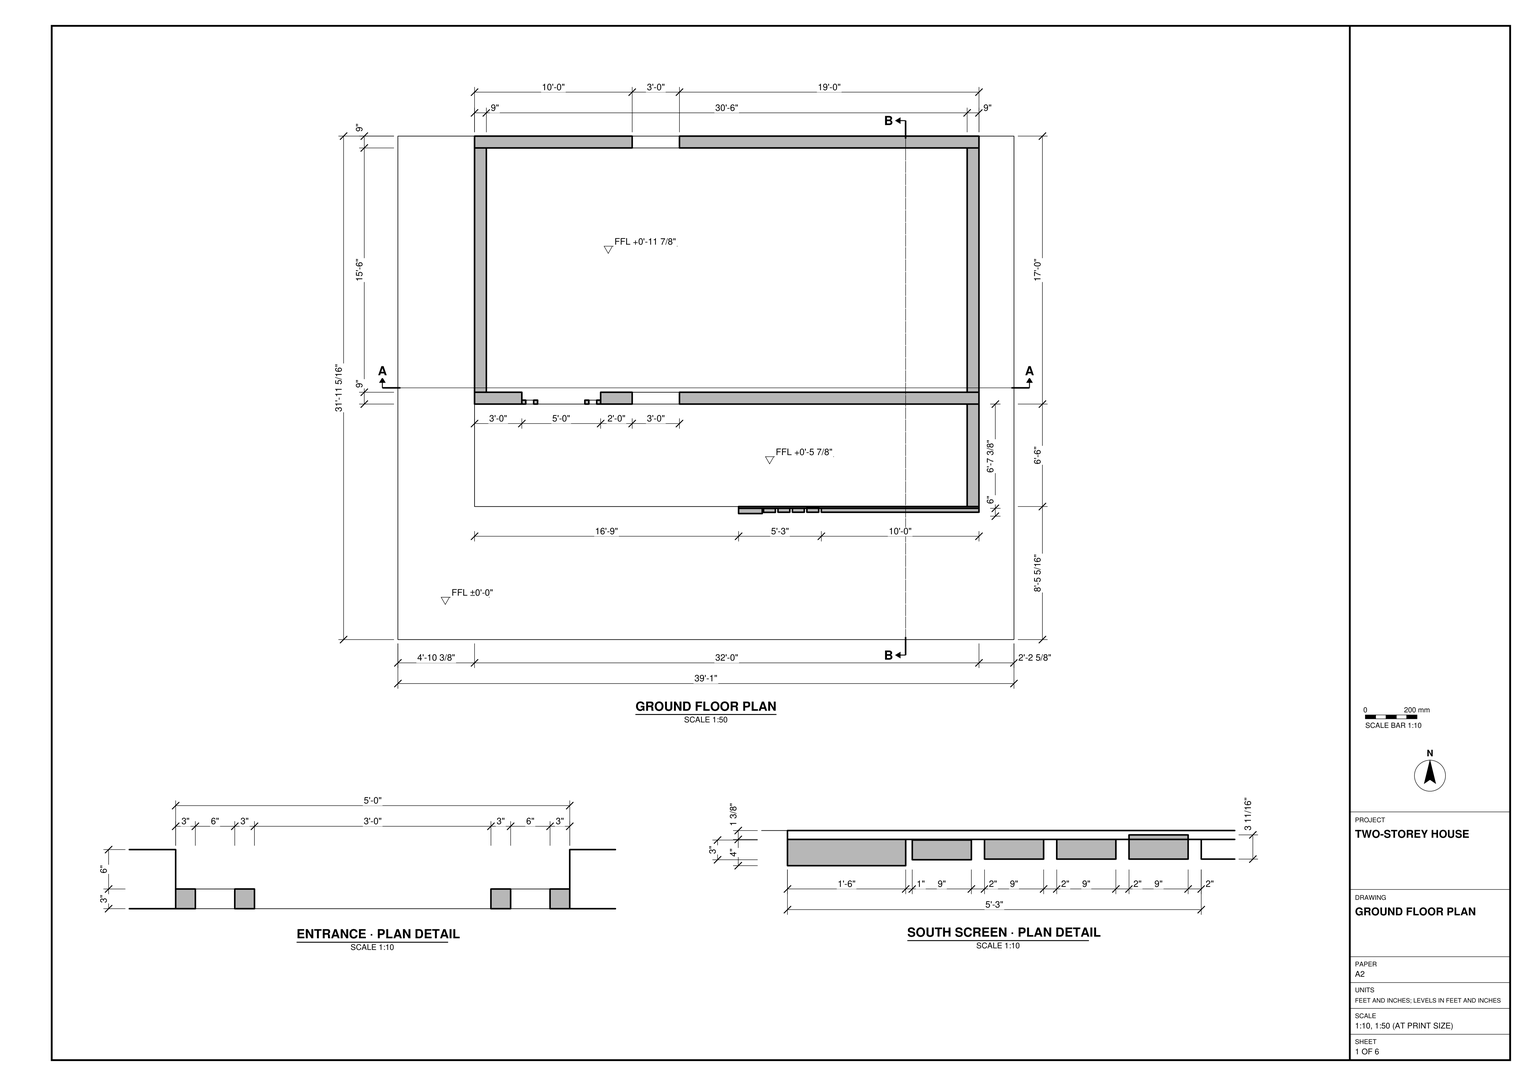
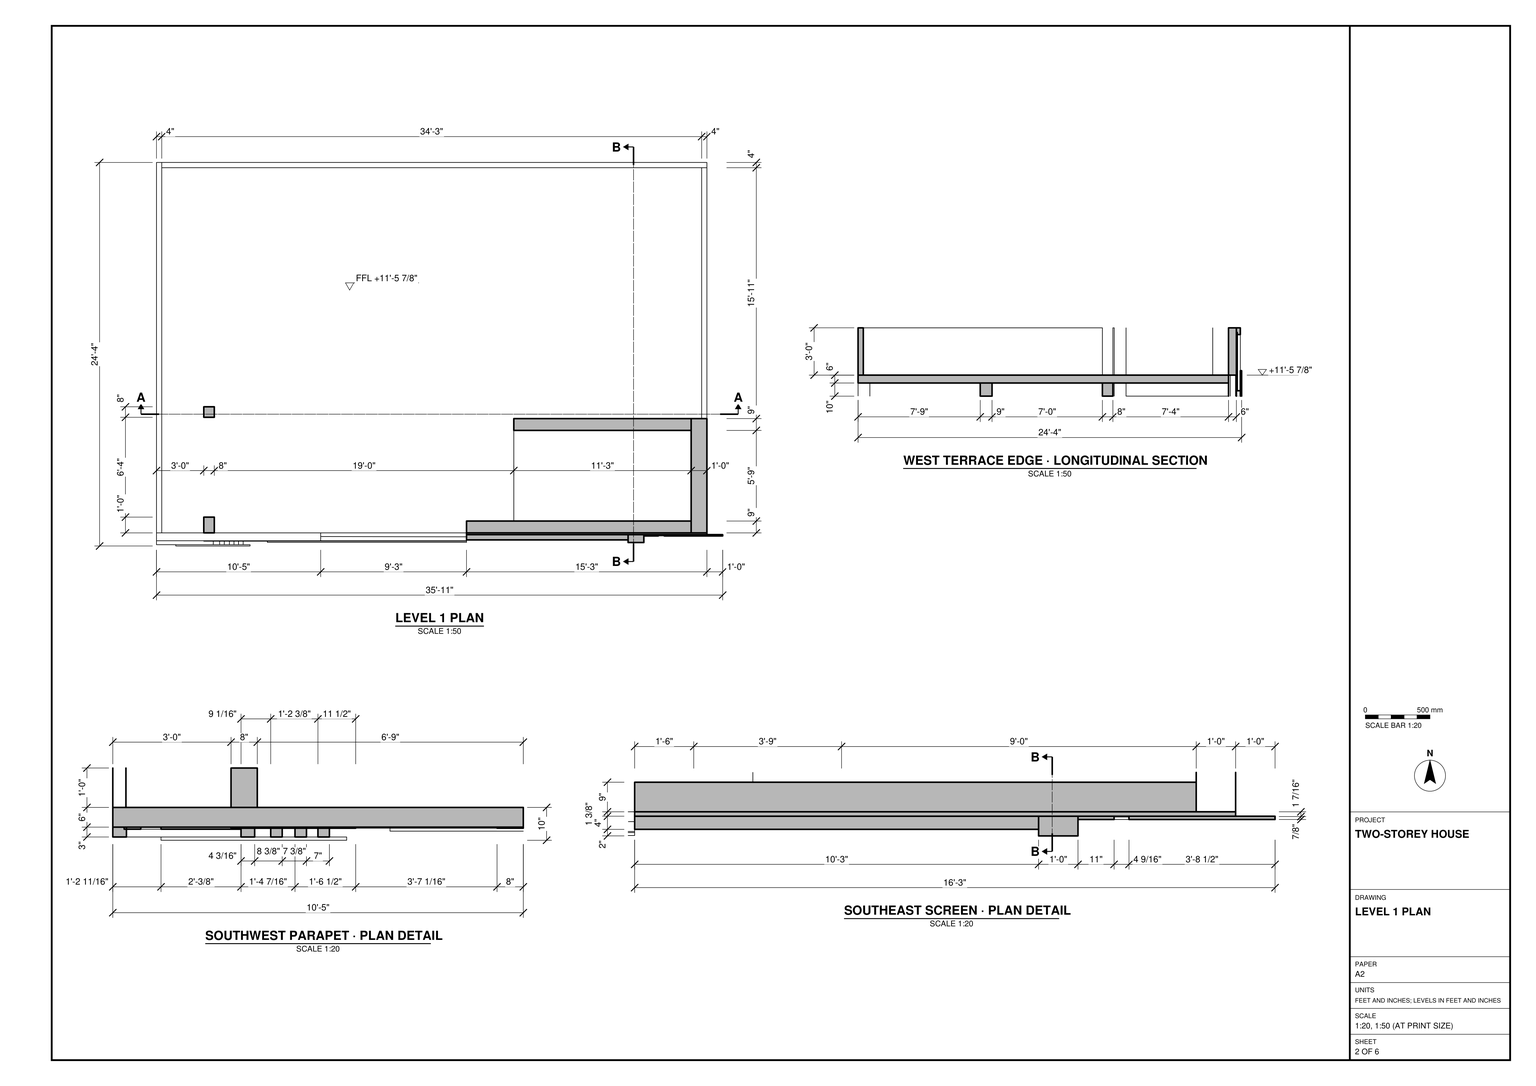
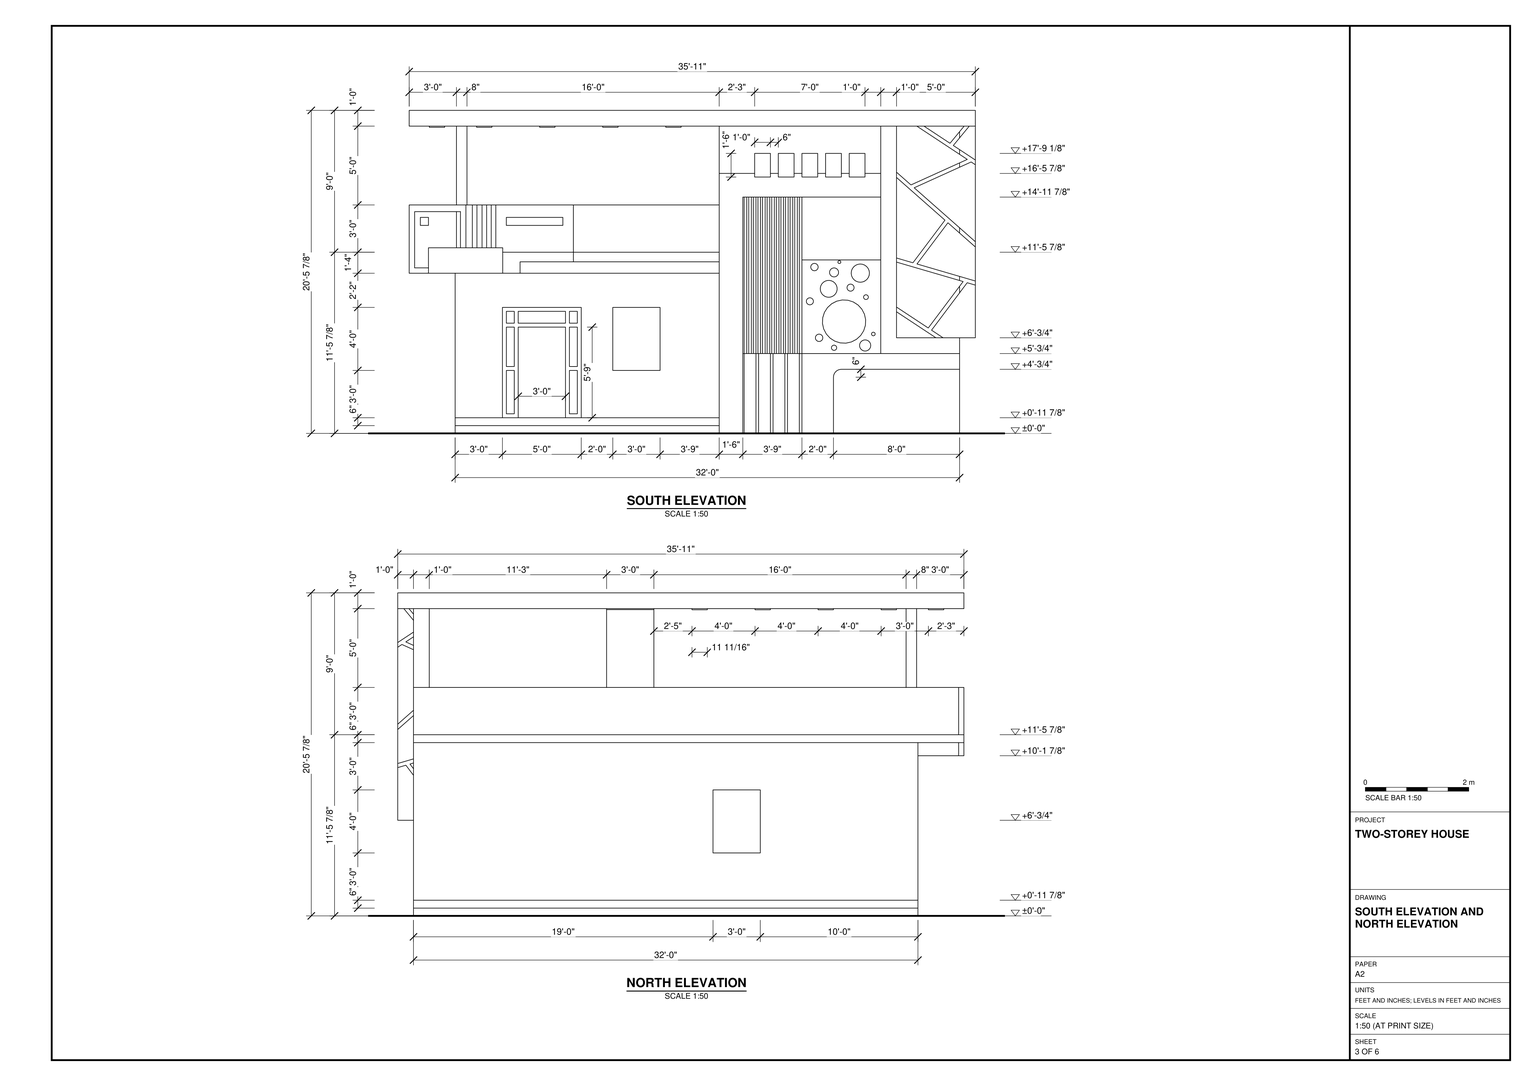
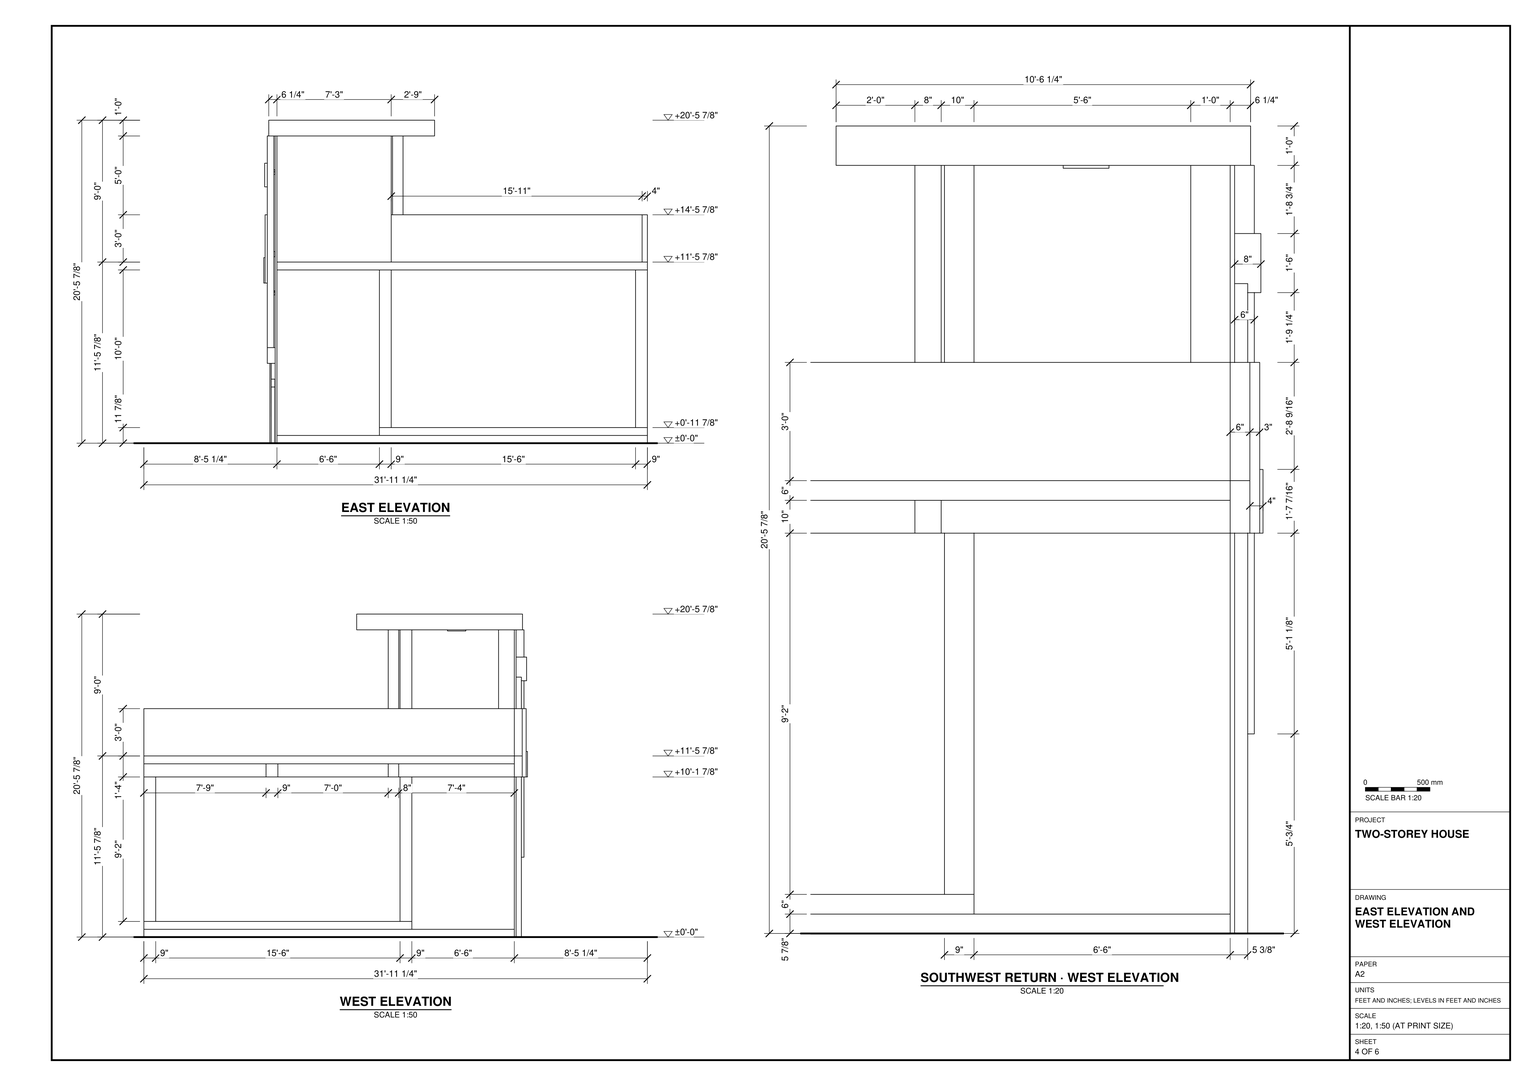
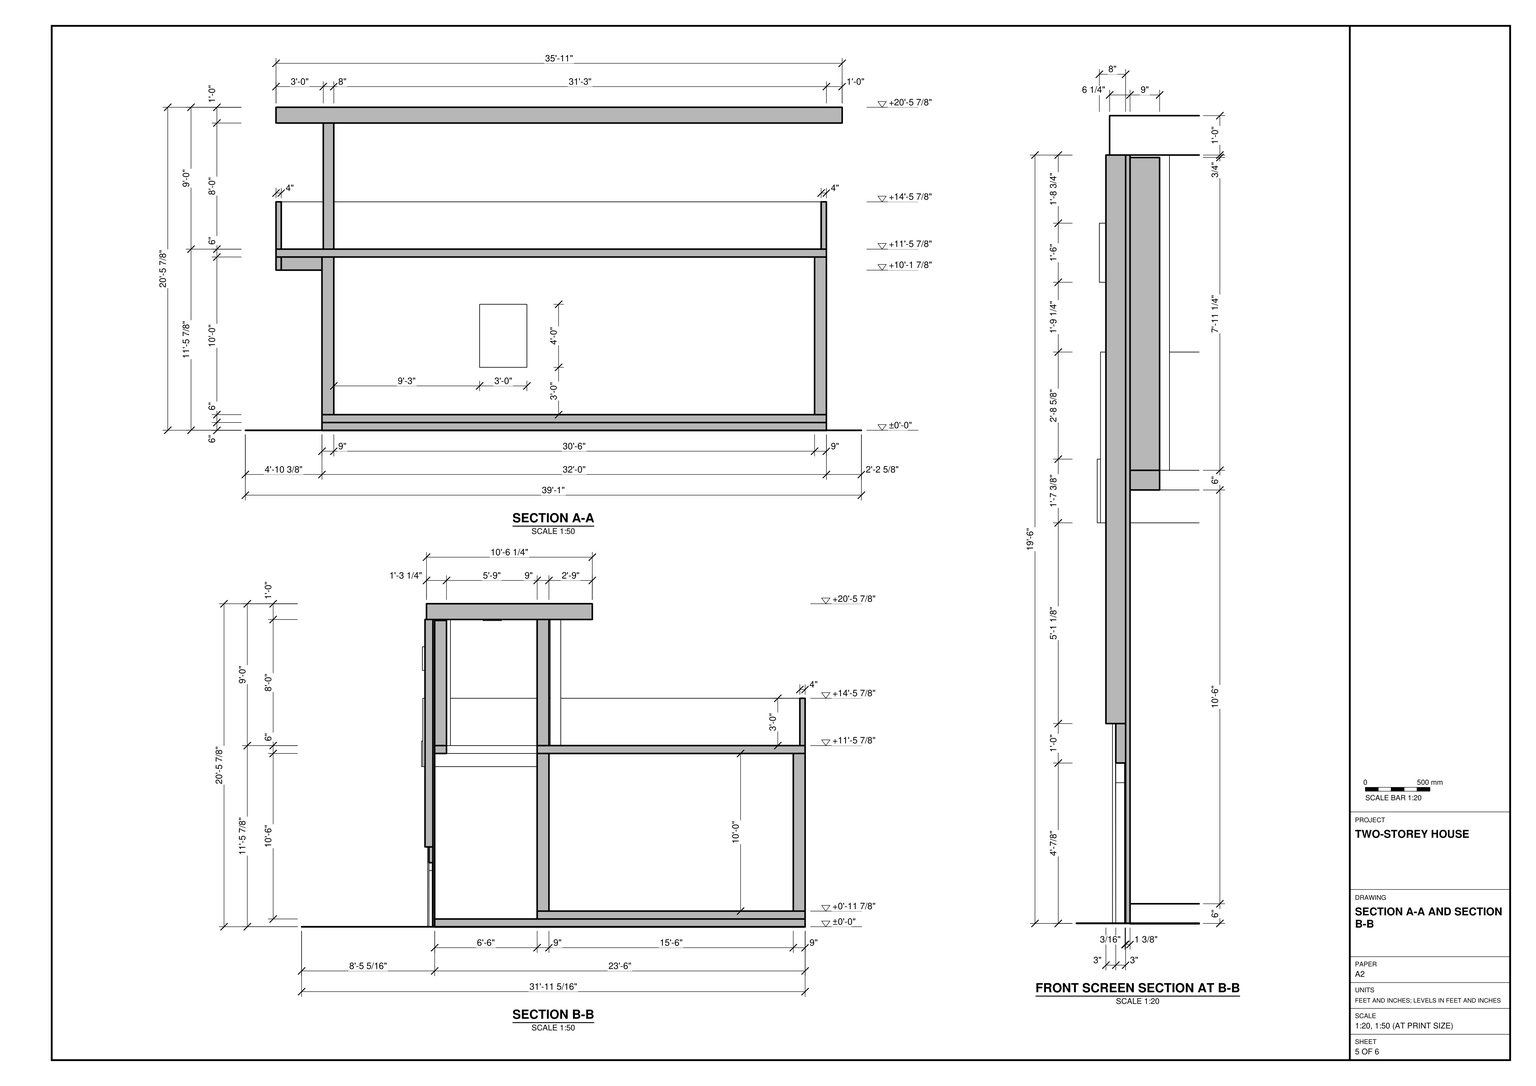
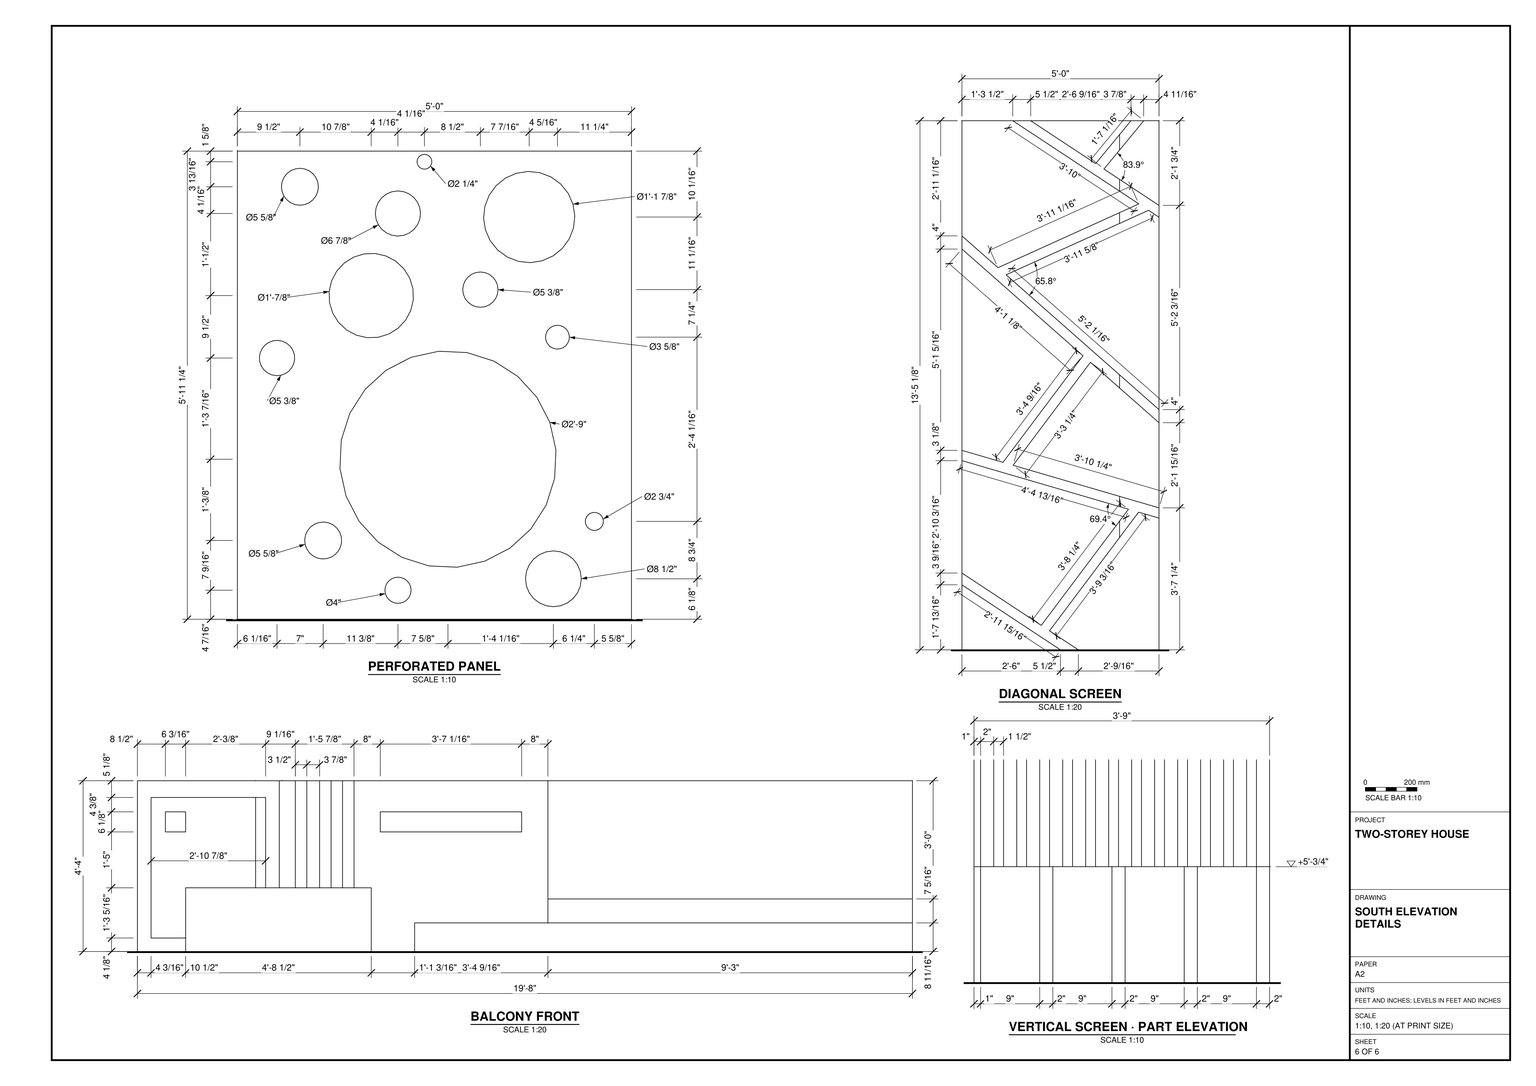
Use task_files/diagram_01.pdf to build the house in SketchUp. Work in feet and inches. Including the base, the model measures 39'-1" along X, 31'-11 5/16" along Y and 20'-6 1/8" along Z. Use ±0'-0" as the ground datum and +11'-5 7/8" as the upper terrace level.

Set out the 32'-0" by 17'-0" ground-floor enclosure on the base with 9" walls. Step up from the base to the south porch at +0'-5 7/8" and then to the interior floor at +0'-11 7/8". Use the entrance detail to frame the doorway, and align the south and north window openings in plan.

Model the projecting terrace slab, its parapets and posts, and the flat roof above. Keep the open space between the parapets and roof as shown in elevation. Use the enlarged plans to set the thickness and spacing of the south screen elements, and the south elevation to place the vertical slats, circular-patterned panel and diagonal end screen.

Keep walls, slabs, roof and individual furniture or joinery pieces in separate groups or components, and use components for repeated parts. Decor and loose items may be any suitable library components. Save one SketchUp model as output_files/two_storey_house_with_covered_terrace_and_south_screens.skp.

# SketchUp Ruby script. Lengths in inches.
U = 1.inch
M = Sketchup.active_model
def pt(a) = Geom::Point3d.new(a.map { |v| v * U })
def face(e, loops, mat)
  f = e.add_face(loops[0].map { |a| pt(a) })
  loops[1..].each { |l| e.add_face(l.map { |a| pt(a) }).erase! }
  f.material = f.back_material = mat if mat
  f
end
# faces: each face lists its corners as indices into pts; further lists are holes
def faces(e, pts, list, mat = nil) = list.each { |f| face(e, (f[0].is_a?(Array) ? f : [f]).map { |l| l.map { |i| pts[i] } }, mat) }
# xy, xz, yz: faces in a plane at the given z, y or x. An outline is a flat list of corners, or four numbers for a rectangle; further outlines are holes
def ring(l) = l.size == 4 ? [[l[0], l[1]], [l[2], l[1]], [l[2], l[3]], [l[0], l[3]]] : l.each_slice(2).to_a
def flat(e, list, mat, &to3) = list.each { |f| face(e, (f[0].is_a?(Array) ? f : [f]).map { |l| ring(l).map { |u, v| to3.(u, v) } }, mat) }
def xy(e, z, list, mat = nil) = flat(e, list, mat) { |x, y| [x, y, z] }
def xz(e, y, list, mat = nil) = flat(e, list, mat) { |x, z| [x, y, z] }
def yz(e, x, list, mat = nil) = flat(e, list, mat) { |y, z| [x, y, z] }
def lines(e, pts, list) = list.each { |a, b| e.add_line(pt(pts[a]), pt(pts[b])) }
# prism: a flat outline (further loops are holes) pulled along v
def prism(e, loops, v, mat = nil)
  f = face(e, loops, mat); d = Geom::Vector3d.new(v.map { |x| x * U })
  f.pushpull(f.normal.samedirection?(d) ? d.length : -d.length)
end
def box(e, o, s, mat = nil) = prism(e, [[o, [o[0] + s[0], o[1], o[2]], [o[0] + s[0], o[1] + s[1], o[2]], [o[0], o[1] + s[1], o[2]]]], [0, 0, s[2]], mat)
def at(x, y, z, deg = 0) = Geom::Transformation.translation(pt([x, y, z])) * Geom::Transformation.rotation(ORIGIN, Z_AXIS, deg.degrees)
def axes(o, x, y, z) = Geom::Transformation.new([*x, 0, *y, 0, *z, 0, *pt(o).to_a, 1])
def part(name) = M.definitions.add(name)
# library, detail: a bought-in or finely detailed component or shape, given as its bounding box
def library(name, o, s) = part(name).tap { |d| box(d.entities, o, s) }
def detail(e, o, s) = box(e.add_group.entities, o, s)
def put(e, d, t, mat = nil) = e.add_instance(d, t).tap { |i| i.material = mat if mat }
def group(e, t, mat = nil) = e.add_group.tap { |g| g.transformation = t; g.material = mat if mat }.entities
root = M.entities
M.materials.add("[0012_Bisque]").color = [255, 228, 196]
M.materials.add("[0072_DarkSeaGreen]").color = [143, 188, 143]
M.materials.add("[0101_CornflowerBlue]").color = [100, 149, 237]
M.materials.add("[Color D05]").color = [255, 191, 0]
M.materials.add("[Color I07]").color = [0, 0, 112]
M.materials.add("[Color M00]").color = [255, 255, 255]
M.materials.add("[Color M05]").color = [114, 114, 114]
M.materials.add("[Color M06]").color = [86, 86, 86]
M.materials.add("[Color M07]").color = [58, 58, 58]
M.materials.add("[Metal Corrugated Shiny]").color = [193, 193, 193]
M.materials.add("[Metal Rusted]").color = [184, 117, 91]
M.materials.add("[Mirror 02]").color = [156, 230, 255]
M.materials["[Mirror 02]"].alpha = 0.29
M.materials.add("[Slate Light Tile]").color = [54, 54, 54]
M.materials.add("[Tile Various Tan]").color = [214, 196, 169]
M.materials.add("[Wood Veneer 01]").color = [120, 70, 37]
c1 = library("Group\#34",[0,-1.8125,0],[60,3,71.27])
c2 = part("Group\#37")
box(c2.entities,[0,0,0],[2,3,119.125])
c3 = part("Group\#45")
xy(c3.entities,0,[[[0,0,11.6875,13.9375],[2.83,2.83,8.86,11.11]]],"[Metal Corrugated Shiny]")
xy(c3.entities,0.625,[[2.83,2.83,8.86,11.11]],"[Metal Rusted]")
xy(c3.entities,0.875,[[[0,0,11.6875,13.9375],[2.83,2.83,8.86,11.11]]])
xz(c3.entities,0,[[0,0,11.6875,0.875]])
xz(c3.entities,2.83,[[2.83,0,8.86,0.625],[2.83,0.625,8.86,0.875]])
xz(c3.entities,11.11,[[2.83,0,8.86,0.625],[2.83,0.625,8.86,0.875]])
xz(c3.entities,13.9375,[[0,0,11.6875,0.875]])
yz(c3.entities,0,[[0,0,13.9375,0.875]])
yz(c3.entities,2.83,[[2.83,0,11.11,0.625],[2.83,0.625,11.11,0.875]])
yz(c3.entities,8.86,[[2.83,0,11.11,0.625],[2.83,0.625,11.11,0.875]])
yz(c3.entities,11.6875,[[0,0,13.9375,0.875]])
xy(root,0,[[0,0,469,383.29]])
xy(root,0.1,[[0,0,469,383.29]],"[Color M00]")
xz(root,0,[[0,0,469,0.1]])
xz(root,383.29,[[0,0,469,0.1]])
yz(root,0,[[0,0,383.29,0.1]])
yz(root,469,[[0,0,383.29,0.1]])
g1 = group(root,at(58.35,-11.09,-24),"[0012_Bisque]")
xy(g1,23.9,[[0,112.375,384,394.375]])
xy(g1,30,[[0,190.375,384,394.375]])
xy(g1,30,[[0,112.375,384,190.375]],"[Slate Light Tile]")
xy(g1,36,[[0,190.375,384,394.375]])
xz(g1,112.375,[[0,23.9,384,30]],"[Slate Light Tile]")
xz(g1,190.375,[[0,30,384,36]],"[Slate Light Tile]")
xz(g1,394.375,[[0,23.9,384,30],[0,30,384,36]])
yz(g1,0,[[112.375,23.9,394.375,30],[190.375,30,394.375,36]])
yz(g1,384,[[112.375,23.9,394.375,30],[190.375,30,394.375,36]])
g2 = group(root,at(58.35,179.29,12),"[0012_Bisque]")
prism(g2,[[[36,9,0],[0,9,0],[0,9,120],[384,9,120],[384,9,0],[96,9,0],[96,9,84],[36,9,84]],[[156,9,84],[120,9,84],[120,9,36],[156,9,36]]],[0,-9,0])
g3 = group(root,at(94.35,179.29,12),"[Wood Veneer 01]")
xy(g3,0,[[0,0,12,3],[48,0,60,3]])
xy(g3,3,[[3,0,9,3],[51,0,57,3]])
xy(g3,36,[[3,0,9,3],[51,0,57,3]])
xy(g3,39,[[3,0,9,3],[51,0,57,3]])
xy(g3,69,[[3,0,9,3],[12,0,48,3],[51,0,57,3]])
xy(g3,72,[[3,0,9,3],[12,0,48,3],[51,0,57,3]])
xy(g3,81,[[3,0,9,3],[12,0,48,3],[51,0,57,3]])
xy(g3,84,[[0,0,60,3]])
xz(g3,0,[[[0,0,12,0,12,69,48,69,48,0,60,0,60,84,0,84],[12,72,48,81],[51,3,57,36],[3,3,9,36],[51,39,57,69],[3,39,9,69],[51,72,57,81],[3,72,9,81]]])
xz(g3,3,[[[0,0,0,84,60,84,60,81,51,81,51,39,57,39,57,81,60,81,60,0,48,0,48,69,12,69,12,0],[12,72,48,81],[51,3,57,36],[3,3,9,36],[3,39,9,69],[3,72,9,81]],[51,69,57,72]])
yz(g3,0,[[0,0,3,84]])
yz(g3,3,[[0,3,3,36],[0,39,3,69],[0,72,3,81]])
yz(g3,9,[[0,3,3,36],[0,39,3,69],[0,72,3,81]])
yz(g3,12,[[0,0,3,69],[0,72,3,81]])
yz(g3,48,[[0,0,3,69],[0,72,3,81]])
yz(g3,51,[[0,3,3,36],[0,39,3,69],[0,72,3,81]])
yz(g3,57,[[0,3,3,36],[0,39,3,69],[0,72,3,81]])
yz(g3,60,[[0,0,3,81],[0,81,3,84]])
g4 = group(root,at(433.35,188.29,12),"[0012_Bisque]")
box(g4,[0,0,0],[9,186,120])
g5 = group(root,at(58.35,374.29,12),"[0012_Bisque]")
prism(g5,[[[384,9,0],[0,9,0],[0,9,120],[384,9,120]],[[156,9,36],[156,9,84],[120,9,84],[120,9,36]]],[0,-9,0])
g6 = group(root,at(58.35,188.29,12),"[0012_Bisque]")
box(g6,[0,0,0],[9,186,120])
g7 = group(root,at(59.35,101.29,120),"[0012_Bisque]")
box(g7,[0,0,2],[8,78,10])
g8 = group(root,at(59.35,101.29,132),"[0012_Bisque]")
prism(g8,[[[383,282,0],[383,0,0],[-36,0,0],[-36,282,0]],[[236,9,0],[371,9,0],[371,78,0],[236,78,0]]],[0,0,6])
g9 = group(root,at(22.35,189.29,120),"[0012_Bisque]")
box(g9,[1,0,2],[35,8,10])
g10 = group(root,at(22.35,281.29,120),"[0012_Bisque]")
box(g10,[1,0,2],[35,9,10])
g11 = group(root,at(23.35,101.29,120),"[0012_Bisque]")
box(g11,[0,0,2],[4,282,10])
g12 = group(root,at(59.35,101.29,138),"[Color M07]")
box(g12,[0,0,0],[8,12,96])
g13 = group(root,at(59.35,189.29,138),"[Color M07]")
box(g13,[0,0,0],[8,8,96])
g14 = group(root,at(430.35,101.29,138),"[0012_Bisque]")
box(g14,[0,0,0],[12,87,96])
g15 = group(root,at(59.35,101.29,234),"[Color M07]")
xy(g15,0,[[-36,-6.23,395,120]],"[0012_Bisque]")
xy(g15,12,[[-36,-6.23,395,120]])
xz(g15,-6.23,[[-36,0,395,12]])
xz(g15,120,[[-36,0,395,12]])
yz(g15,-36,[[-6.23,0,120,12]])
yz(g15,395,[[-6.23,0,120,12]])
g16 = group(root,at(23.35,95.29,126),"[0012_Bisque]")
box(g16,[0,0,-4],[236,6,16])
g17 = group(root,at(23.35,95.29,138),"[0012_Bisque]")
box(g17,[0,0,0],[125,6,36])
g18 = group(root,at(23.35,92.29,138),"[0101_CornflowerBlue]")
prism(g18,[[[0,0,-16],[43.2,0,-16],[43.2,0,36],[0,0,36]],[[4.16,0,30.9],[39.04,0,30.9],[39.04,0,-11.9],[4.16,0,-11.9]]],[0,3,0])
g19 = group(root,at(26.82,94.29,141.47),"[0072_DarkSeaGreen]")
prism(g19,[[[0,1,-15.36],[0,1,29.07],[35.58,1,29.07],[35.58,1,-15.36]],[[11.22,1,23.07],[5.05,1,23.07],[5.05,1,16.95],[11.22,1,16.95]]],[0,-0.63,0])
g20 = group(root,at(71.4375,92.29,138),"[Color M07]")
box(g20,[0,0,-16],[3.5,3,52])
g21 = group(root,at(78.83,92.29,138),"[Color M07]")
box(g21,[0,0,-16],[3.5,3,52])
g22 = group(root,at(85.81,92.29,138),"[Color M07]")
box(g22,[0,0,-16],[3.5,3,52])
g23 = group(root,at(38.04,91.29,121),"[Color D05]")
box(g23,[0,0,1],[56.52,1,19.4])
g24 = group(root,at(59.35,95.09,122))
xy(g24,0,[[0,-0.125,200,0.2]],"[0012_Bisque]")
xy(g24,16,[[89,-0.125,200,0.2]],"[0012_Bisque]")
xy(g24,36.42,[[37.96,-0.125,81,0.2]],"[0012_Bisque]")
xy(g24,42.53,[[37.96,-0.125,81,0.2]],"[0012_Bisque]")
xy(g24,52,[[0,-0.125,89,0.2]],"[0012_Bisque]")
xz(g24,-0.125,[[89,0,200,16]],"[0012_Bisque]")
xz(g24,-0.125,[[[0,0,89,52],[37.96,36.42,81,42.53]]],"[Color M05]")
xz(g24,0.2,[[[0,0,0,52,89,52,89,16,200,16,200,0],[37.96,36.42,81,42.53]]],"[0012_Bisque]")
yz(g24,0,[[-0.125,0,0.2,52]],"[0012_Bisque]")
yz(g24,37.96,[[-0.125,36.42,0.2,42.53]],"[0012_Bisque]")
yz(g24,81,[[-0.125,36.42,0.2,42.53]],"[0012_Bisque]")
yz(g24,89,[[-0.125,16,0.2,52]],"[0012_Bisque]")
yz(g24,200,[[-0.125,0,0.2,16]],"[0012_Bisque]")
g25 = group(root,at(107.77,94.0625,122),"[0072_DarkSeaGreen]")
box(g25,[0,0,0],[151.59,1,8.7])
g26 = group(root,at(295.35,179.29,138),"[0012_Bisque]")
box(g26,[0,0,0],[135,9,96])
g27 = group(root,at(259.35,101.29,138),"[0012_Bisque]")
box(g27,[0,0,0],[171,9,95.25])
g28 = group(root,at(259.35,99.9375,0),"[0012_Bisque]")
box(g28,[0,0,0],[183,1.35,234])
g29 = group(root,at(394.35,98.9375,72.875))
xy(g29,0,[[0,0,30,1],[35.45,0,60,1],[30,0.9,35.45,1]])
xy(g29,161.125,[[0,0,15.47,1],[20.92,0,51.47,1],[55.36,0,60,1],[15.47,0.9,20.92,1],[51.47,0.9,55.36,1]])
xz(g29,0,[[0,0,30,0,0,19.79],[35.45,0,60,0,60,40.11,53.78,41.93,26.66,5.8],[24.15,7.45,50.71,42.83,0,57.62,0,23.38],[60,43.24,60,69.16,39.12,87.5625,15.57,56.2],[12.49,57.1,36.86,89.55,0,122.06,0,60.74],
  [60,73.16,60,131.75,56.82,133.85,13.45,114.2],[10.98,116.375,53.86,135.8,38.79,145.74,15.47,161.125,0,161.125,0,126.06],[60,135.35,60,161.125,55.36,161.125,43.23,146.41],[40.71,148.07,51.47,161.125,20.92,161.125]],"[Color M06]")
xz(g29,0.9,[[30,0,35.45,0,26.66,5.8,53.78,41.93,60,40.11,60,43.24,15.57,56.2,39.12,87.5625,60,69.16,60,73.16,13.45,114.2,56.82,133.85,60,131.75,60,135.35,43.23,146.41,55.36,161.125,51.47,161.125,40.71,148.07,20.92,161.125,15.47,161.125,38.79,145.74,53.86,135.8,10.98,116.375,0,126.06,0,122.06,36.86,89.55,12.49,57.1,0,60.74,0,57.62,50.71,42.83,24.15,7.45,0,23.38,0,19.79]])
xz(g29,1,[[0,0,0,19.79,30,0],[35.45,0,26.66,5.8,53.78,41.93,60,40.11,60,0],[24.15,7.45,0,23.38,0,57.62,50.71,42.83],[60,43.24,15.57,56.2,39.12,87.5625,60,69.16],[12.49,57.1,0,60.74,0,122.06,36.86,89.55],
  [60,73.16,13.45,114.2,56.82,133.85,60,131.75],[10.98,116.375,0,126.06,0,161.125,15.47,161.125,38.79,145.74,53.86,135.8],[60,135.35,43.23,146.41,55.36,161.125,60,161.125],[40.71,148.07,20.92,161.125,51.47,161.125]])
yz(g29,0,[[0,0,1,19.79],[0.9,19.79,1,23.38],[0,23.38,1,57.62],[0.9,57.62,1,60.74],[0,60.74,1,122.06],
  [0.9,122.06,1,126.06],[0,126.06,1,161.125]])
yz(g29,60,[[0,0,1,40.11],[0.9,40.11,1,43.24],[0,43.24,1,69.16],[0.9,69.16,1,73.16],[0,73.16,1,131.75],
  [0.9,131.75,1,135.35],[0,135.35,1,161.125]])
p = [[0,0,19.79],[30,0,0],[30,0.9,0],[0,0.9,19.79],[35.45,0,0],[26.66,0,5.8],
  [26.66,0.9,5.8],[35.45,0.9,0],[30,1,0],[0,1,19.79],[26.66,1,5.8],[35.45,1,0],
  [53.78,0,41.93],[53.78,0.9,41.93],[53.78,1,41.93],[24.15,0,7.45],[0,0,23.38],[0,0.9,23.38],
  [24.15,0.9,7.45],[50.71,0,42.83],[50.71,0.9,42.83],[0,1,23.38],[24.15,1,7.45],[50.71,1,42.83],
  [60,0,40.11],[60,0.9,40.11],[60,1,40.11],[0,0,57.62],[0,0.9,57.62],[0,1,57.62],
  [60,0,43.24],[15.57,0,56.2],[15.57,0.9,56.2],[60,0.9,43.24],[15.57,1,56.2],[60,1,43.24],
  [39.12,0,87.5625],[39.12,0.9,87.5625],[39.12,1,87.5625],[12.49,0,57.1],[0,0,60.74],[0,0.9,60.74],
  [12.49,0.9,57.1],[36.86,0,89.55],[36.86,0.9,89.55],[0,1,60.74],[12.49,1,57.1],[36.86,1,89.55],
  [60,0,69.16],[60,0.9,69.16],[60,1,69.16],[60,0,73.16],[13.45,0,114.2],[13.45,0.9,114.2],
  [60,0.9,73.16],[13.45,1,114.2],[60,1,73.16],[0,0,122.06],[0,0.9,122.06],[0,1,122.06],
  [56.82,0,133.85],[56.82,0.9,133.85],[56.82,1,133.85],[10.98,0,116.375],[0,0,126.06],[0,0.9,126.06],
  [10.98,0.9,116.375],[53.86,0,135.8],[53.86,0.9,135.8],[0,1,126.06],[10.98,1,116.375],[53.86,1,135.8],
  [60,0,131.75],[60,0.9,131.75],[60,1,131.75],[60,0,135.35],[43.23,0,146.41],[43.23,0.9,146.41],
  [60,0.9,135.35],[43.23,1,146.41],[60,1,135.35],[38.79,0,145.74],[38.79,0.9,145.74],[38.79,1,145.74],
  [15.47,0,161.125],[15.47,0.9,161.125],[15.47,1,161.125],[55.36,0,161.125],[55.36,0.9,161.125],[55.36,1,161.125],
  [40.71,0,148.07],[20.92,0,161.125],[20.92,0.9,161.125],[40.71,0.9,148.07],[51.47,0,161.125],[51.47,0.9,161.125],
  [20.92,1,161.125],[40.71,1,148.07],[51.47,1,161.125]]
faces(g29,p,[[0,1,2,3],[4,5,6,7],[8,9,3,2],[10,11,7,6],[5,12,13,6],[14,10,6,13],[15,16,17,18],[19,15,18,20],
  [21,22,18,17],[22,23,20,18],[12,24,25,13],[26,14,13,25],[27,19,20,28],[23,29,28,20],[30,31,32,33],[34,35,33,32],
  [31,36,37,32],[38,34,32,37],[39,40,41,42],[43,39,42,44],[45,46,42,41],[46,47,44,42],[36,48,49,37],[50,38,37,49],
  [51,52,53,54],[55,56,54,53],[57,43,44,58],[47,59,58,44],[52,60,61,53],[62,55,53,61],[63,64,65,66],[67,63,66,68],
  [69,70,66,65],[70,71,68,66],[60,72,73,61],[74,62,61,73],[75,76,77,78],[79,80,78,77],[81,67,68,82],[71,83,82,68],
  [84,81,82,85],[83,86,85,82],[76,87,88,77],[89,79,77,88],[90,91,92,93],[94,90,93,95],[96,97,93,92],[97,98,95,93]])
g30 = group(root,at(322.35,93.9375,0),"[Color M05]")
xy(g30,0,[[0,3,24,6]])
xy(g30,48.875,[[30,3,120,6]])
xy(g30,60.875,[[60,0,120,3],[0,3,60,6],[60,3,120,6]])
xy(g30,72.875,[[72,0,120,6]])
xy(g30,234,[[60,0,72,6]])
xz(g30,0,[[60,60.875,120,60.875,120,72.875,72,72.875,72,234,60,234]],"[Color M00]")
xz(g30,3,[[0,0,24,0,24,42.875,24.05,43.66,24.2,44.43,24.46,45.17,24.8,45.875,25.24,46.53,25.76,47.12,26.35,47.64,27,48.07,27.7,48.42,28.45,48.67,29.22,48.82,30,48.875,120,48.875,120,60.875,0,60.875]],"[Color M06]")
xz(g30,6,[[0,0,0,60.875,120,60.875,120,48.875,30,48.875,29.22,48.82,28.45,48.67,27.7,48.42,27,48.07,26.35,47.64,25.76,47.12,25.24,46.53,24.8,45.875,24.46,45.17,24.2,44.43,24.05,43.66,24,42.875,24,0],[60,60.875,60,234,72,234,72,72.875,120,72.875,120,60.875]])
yz(g30,0,[[3,0,6,60.875]])
yz(g30,24,[[3,0,6,42.875]])
yz(g30,60,[[0,60.875,6,234]])
yz(g30,72,[[0,72.875,6,234]])
yz(g30,120,[[3,48.875,6,60.875],[0,60.875,6,72.875]])
p = [[24,6,42.875],[24.05,6,43.66],[24.05,3,43.66],[24,3,42.875],[24.2,6,44.43],[24.2,3,44.43],
  [24.46,6,45.17],[24.46,3,45.17],[24.8,6,45.875],[24.8,3,45.875],[25.24,6,46.53],[25.24,3,46.53],
  [25.76,6,47.12],[25.76,3,47.12],[26.35,6,47.64],[26.35,3,47.64],[27,6,48.07],[27,3,48.07],
  [27.7,6,48.42],[27.7,3,48.42],[28.45,6,48.67],[28.45,3,48.67],[29.22,6,48.82],[29.22,3,48.82],
  [30,6,48.875],[30,3,48.875]]
faces(g30,p,[[0,1,2,3],[1,4,5,2],[4,6,7,5],[6,8,9,7],[8,10,11,9],[10,12,13,11],[12,14,15,13],[14,16,17,15],
  [16,18,19,17],[18,20,21,19],[20,22,23,21],[22,24,25,23]])
g31 = group(root,at(346.35,99.74,0),"[Tile Various Tan]")
prism(g31,[[[0,0.2,0],[0,0.2,42.875],[0.05,0.2,43.66],[0.2,0.2,44.43],[0.46,0.2,45.17],[0.8,0.2,45.875],[1.24,0.2,46.53],[1.76,0.2,47.12],[2.35,0.2,47.64],[3,0.2,48.07],[3.7,0.2,48.42],[4.45,0.2,48.67],[5.22,0.2,48.82],[6,0.2,48.875],[96,0.2,48.875],[96,0.2,0]]],[0,-0.2,0])
g32 = group(root,at(259.35,95.9375,0),"[Color M07]")
prism(g32,[[[18,4,180],[18,4,0],[0,4,0],[0,4,198],[123,4,198],[123,4,180]]],[0,-4,0])
g33 = group(root,at(286.35,91.9375,195.25),"[Color D05]")
box(g33,[18,0,0],[12,8,18])
box(g33,[0,0,0],[12,8,18])
box(g33,[54,0,0],[12,8,18])
box(g33,[36,0,0],[12,8,18])
box(g33,[72,0,0],[12,8,18])
put(root,c1,at(322.35,98.75,60.875))
g34 = group(root,at(322.35,99.84,132.15),"[0012_Bisque]")
box(g34,[0,0,0],[60,0.1,47.85])
g35 = group(root,at(277.35,99.84,60.875),"[Color I07]")
box(g35,[0,0,0],[45,0.1,119.125])
g36 = group(root,at(278.35,96.84,60.875),"[0101_CornflowerBlue]")
put(g36,c2,at(28,0,0))
put(g36,c2,at(14,0,0))
put(g36,c2,at(24.5,0,0))
put(g36,c2,at(3.5,0,0))
put(g36,c2,at(7,0,0))
put(g36,c2,at(35,0,0))
put(g36,c2,at(0,0,0))
put(g36,c2,at(38.5,0,0))
put(g36,c2,at(42,0,0))
put(g36,c2,at(21,0,0))
put(g36,c2,at(10.5,0,0))
put(g36,c2,at(17.5,0,0))
put(g36,c2,at(31.5,0,0))
g37 = group(root,at(278.35,96.84,0),"[0012_Bisque]")
box(g37,[11,0.1,0],[9,3,60.88])
box(g37,[22,0.1,0],[9,3,60.88])
prism(g37,[[[0,3.1,0],[9,3.1,0],[9,0.1,0],[0,0.1,0]]],[0,-0.1,60.875])
box(g37,[33,0.1,0],[9,3.69,60.88])
g38 = group(root,at(433.35,101.29,12),"[0012_Bisque]")
box(g38,[0,0,-6],[9,78,126])
g39 = group(root,at(23.35,101.29,138),"[0012_Bisque]")
box(g39,[0,0,0],[4,282,36])
g40 = group(root,at(27.35,379.29,138),"[0012_Bisque]")
box(g40,[0,0,0],[415,4,36])
g41 = group(root,at(438.35,188.29,138),"[0012_Bisque]")
box(g41,[0,0,0],[4,191,36])
g42 = group(root,at(148.35,98.29,138),"[Mirror 02]")
p = [[0,0.23,0],[0,0.23,36],[111,0,36],[111,0,0]]
faces(g42,p,[[0,1,2,3]])
put(root,c3,at(218.68,138.19,233.125))
put(root,c3,at(170.68,138.19,233.125))
put(root,c3,at(122.68,138.19,233.125))
put(root,c3,at(74.68,138.19,233.125))
put(root,c3,at(38.68,138.19,233.125))
